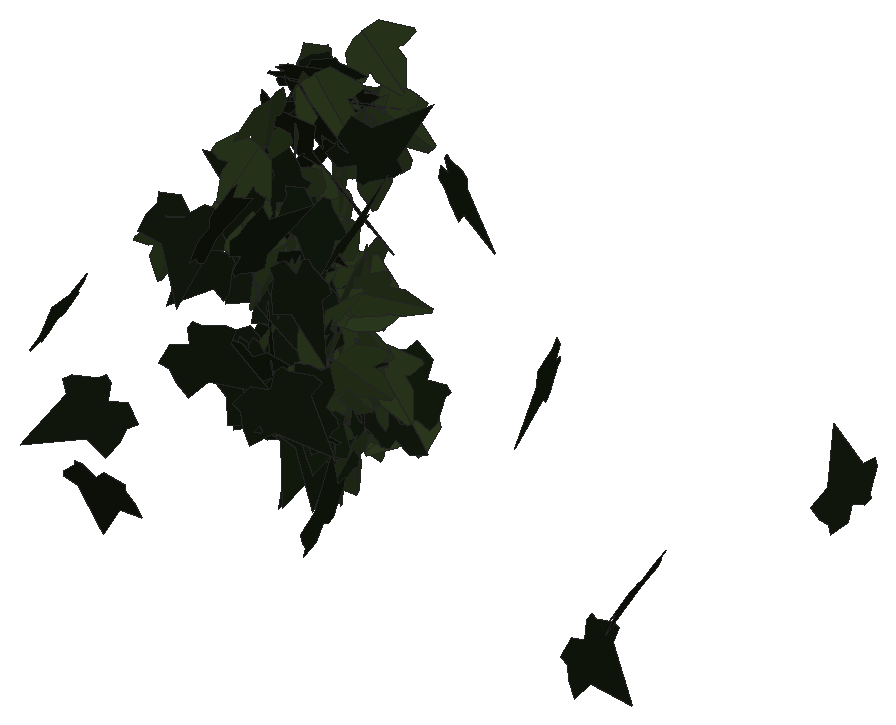
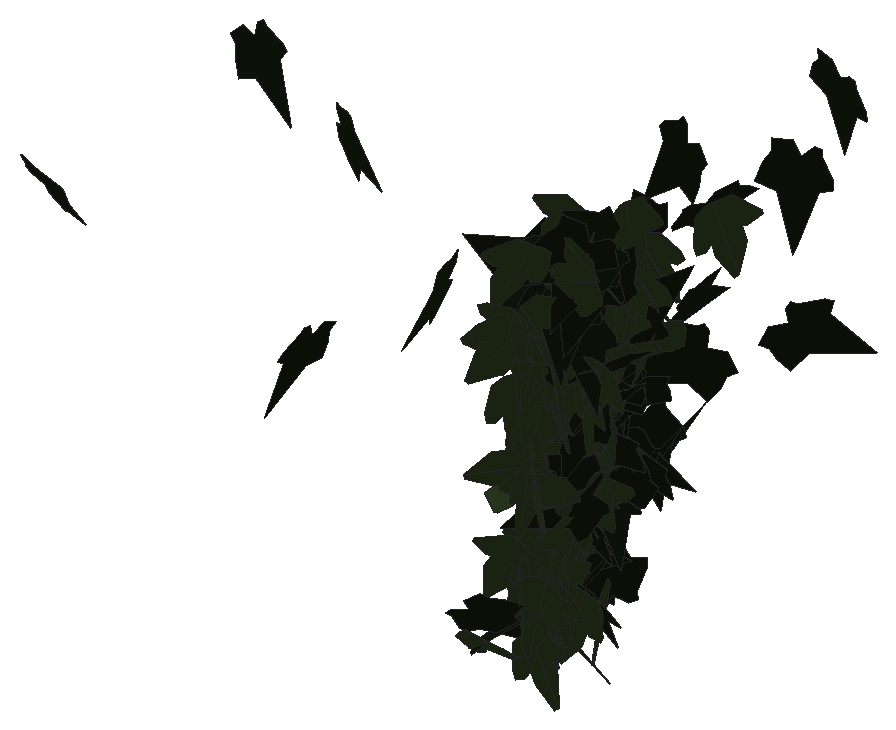
# SketchUp Ruby script. Lengths in inches.
U = 1.inch
M = Sketchup.active_model
def pt(a) = Geom::Point3d.new(a.map { |v| v * U })
def face(e, loops, mat)
  f = e.add_face(loops[0].map { |a| pt(a) })
  loops[1..].each { |l| e.add_face(l.map { |a| pt(a) }).erase! }
  f.material = f.back_material = mat if mat
  f
end
# faces: each face lists its corners as indices into pts; further lists are holes
def faces(e, pts, list, mat = nil) = list.each { |f| face(e, (f[0].is_a?(Array) ? f : [f]).map { |l| l.map { |i| pts[i] } }, mat) }
# xy, xz, yz: faces in a plane at the given z, y or x. An outline is a flat list of corners, or four numbers for a rectangle; further outlines are holes
def ring(l) = l.size == 4 ? [[l[0], l[1]], [l[2], l[1]], [l[2], l[3]], [l[0], l[3]]] : l.each_slice(2).to_a
def flat(e, list, mat, &to3) = list.each { |f| face(e, (f[0].is_a?(Array) ? f : [f]).map { |l| ring(l).map { |u, v| to3.(u, v) } }, mat) }
def xy(e, z, list, mat = nil) = flat(e, list, mat) { |x, y| [x, y, z] }
def xz(e, y, list, mat = nil) = flat(e, list, mat) { |x, z| [x, y, z] }
def yz(e, x, list, mat = nil) = flat(e, list, mat) { |y, z| [x, y, z] }
def lines(e, pts, list) = list.each { |a, b| e.add_line(pt(pts[a]), pt(pts[b])) }
# prism: a flat outline (further loops are holes) pulled along v
def prism(e, loops, v, mat = nil)
  f = face(e, loops, mat); d = Geom::Vector3d.new(v.map { |x| x * U })
  f.pushpull(f.normal.samedirection?(d) ? d.length : -d.length)
end
def box(e, o, s, mat = nil) = prism(e, [[o, [o[0] + s[0], o[1], o[2]], [o[0] + s[0], o[1] + s[1], o[2]], [o[0], o[1] + s[1], o[2]]]], [0, 0, s[2]], mat)
def at(x, y, z, deg = 0) = Geom::Transformation.translation(pt([x, y, z])) * Geom::Transformation.rotation(ORIGIN, Z_AXIS, deg.degrees)
def axes(o, x, y, z) = Geom::Transformation.new([*x, 0, *y, 0, *z, 0, *pt(o).to_a, 1])
def part(name) = M.definitions.add(name)
# library, detail: a bought-in or finely detailed component or shape, given as its bounding box
def library(name, o, s) = part(name).tap { |d| box(d.entities, o, s) }
def detail(e, o, s) = box(e.add_group.entities, o, s)
def put(e, d, t, mat = nil) = e.add_instance(d, t).tap { |i| i.material = mat if mat }
def group(e, t, mat = nil) = e.add_group.tap { |g| g.transformation = t; g.material = mat if mat }.entities
root = M.entities
M.materials.add("efeu1").color = [18, 25, 13]
M.materials.add("efeu2").color = [43, 57, 29]
c1 = part("ivyleaf_10")
p = [[0,0.5,-0.03],[-0.0625,2.02,-0.43],[-0.19,2.01,-0.46],[-0.54,1.05,-0.29],[-0.52,0.625,-0.18],[-0.83,0.76,-0.28],
  [-1.16,0.64,-0.33],[-1.15,0.33,-0.24],[-0.77,-0.39,0.02],[-0.3,-0.51,0.16],[0.04,-0.48,0.23],[-0.02,2.01,-0.4375],
  [-0.06,2.01,-0.43],[0.04,-0.49,0.23],[0.67,-0.49,0.14],[1.38,0.36,-0.2],[1.375,0.51,-0.24],[0.81,0.65,-0.19],
  [0.62,0.59,-0.15],[0.6,1.09,-0.28],[0.5,1.23,-0.31]]
faces(c1.entities,p,[[0,1,2,3,4,5,6,7,8,9,10],[11,12,0,13,14,15,16,17,18,19,20]],"efeu2")
c2 = part("ivyleaf_9")
p = [[1.54,2.16,1.25],[1.36,2.04,1.19],[-0.21,0.99,0.68],[-0.71,1.11,0.82],[-0.85,0.86,0.67],[-0.8,0.17,0.21],
  [-0.9,-0.01,0.1],[-0.67,-0.16,-0.02],[-0.08,-0.08,-0.05],[-0.03,-0.6,-0.4],[0.65,-0.88,-0.66],[0.83,-0.6,-0.49],
  [1.29,-0.42,-0.43],[1.8125,-0.07,-0.26],[1.21,0.44,0.15]]
faces(c2.entities,p,[[0,1,2,3,4,5,6,7,8,9,10,11,12,13,14]],"efeu1")
put(root,c1,axes([54.52,225.38,209.37],[0.06794,0.47554,0.13874],[-0.053,0.14622,-0.4752],[-0.49252,0.04986,0.07027]))
put(root,c2,axes([54.43,224.8,212.04],[-0.17029,-0.46723,0.05192],[0.09679,-0.08888,-0.48242],[0.46004,-0.15425,0.12071]))
put(root,c1,axes([54.47,224.94,211.95],[-0.46815,-0.03134,-0.17279],[0.17195,-0.18173,-0.43291],[-0.03567,-0.46475,0.18093]))
put(root,c1,axes([54.58,224.75,211.125],[0.07251,-0.48194,0.11169],[0.03199,-0.10808,-0.48713],[0.49368,0.07778,0.01516]))
put(root,c1,axes([54.57,224.875,209.74],[0.11655,0.09989,-0.47586],[0.0633,0.48205,0.1167],[0.48209,-0.08745,0.09972]))
put(root,c2,axes([54.8,219.61,210.4],[-0.01506,-0.06036,-0.49611],[-0.11412,-0.48281,0.06221],[-0.48657,0.11511,0.00076]))
put(root,c1,axes([54.61,223.75,213.02],[-0.18239,-0.43215,-0.17316],[0.0597,0.16273,-0.46899],[0.4617,-0.19175,-0.00776]))
put(root,c1,axes([54.76,224.34,207.58],[-0.23006,0.25819,0.36112],[-0.24578,0.26463,-0.34578],[-0.36969,-0.33661,0.00515]))
put(root,c2,axes([54.84,223.76,212.22],[0.08417,0.02553,0.4922],[-0.48104,-0.10448,0.08767],[0.10733,-0.48829,0.00697]))
put(root,c1,axes([54.66,224.65,209.55],[-0.47194,0.16379,0.02103],[-0.0203,0.00564,-0.49956],[-0.16388,-0.47238,0.00132]))
put(root,c2,axes([54.83,224.15,209.55],[-0.10043,0.48531,0.06627],[-0.03715,0.05991,-0.49501],[-0.4884,-0.10435,0.02402]))
put(root,c1,axes([54.67,226.05,208.43],[-0.49533,0.06801,0.00507],[-0.00501,0.00076,-0.49997],[-0.06801,-0.49535,-0.00007]))
put(root,c1,axes([54.95,225.86,207.34],[-0.39652,0.03395,0.30269],[-0.30458,-0.04808,-0.3936],[0.00238,-0.49652,0.05881]))
put(root,c2,axes([54.87,224.76,212.64],[-0.07203,0.48635,-0.09095],[0.01821,-0.08924,-0.49163],[-0.49445,-0.07413,-0.00485]))
put(root,c2,axes([54.4,225.17,209.96],[0.44623,0.05922,0.21766],[0.20549,0.09228,-0.44638],[-0.09304,0.48783,0.05802]))
put(root,c1,axes([54.73,225.03,207.79],[-0.49219,0.06307,-0.06142],[0.06021,-0.01334,-0.49618],[-0.06423,-0.49583,0.00554]))
put(root,c1,axes([54.85,225.43,212.1],[0.29412,-0.27482,-0.29659],[-0.15217,0.26457,-0.39604],[0.37462,0.32323,0.07199]))
put(root,c2,axes([54.62,224.63,211.08],[-0.07419,-0.47381,0.14143],[0.00295,-0.14344,-0.47897],[0.49446,-0.07024,0.02407]))
put(root,c2,axes([54.97,224.75,213.92],[-0.45932,0.18416,-0.07144],[0.05499,-0.05447,-0.49397],[-0.18973,-0.46165,0.02979]))
put(root,c1,axes([54.89,224.2,212.43],[-0.32114,-0.36465,0.11788],[-0.08489,-0.08229,-0.48582],[0.37371,-0.33205,-0.00906]))
put(root,c2,axes([54.82,224.61,213.58],[0.20655,0.45525,0.00906],[-0.01589,0.01715,-0.49945],[-0.45507,0.20603,0.02155]))
put(root,c1,axes([54.4,225.23,213.76],[0.1666,-0.04389,0.46938],[0.46109,0.11885,-0.15255],[-0.09818,0.48368,0.08008]))
put(root,c1,axes([54.8125,224.56,209.5],[0.35481,0.28865,-0.20197],[-0.15364,-0.13117,-0.45737],[-0.31703,0.38662,-0.00438]))
put(root,c1,axes([54.64,223.17,211.71],[0.40941,0.21968,-0.18472],[0.15871,0.09485,0.46456],[0.23915,-0.43902,0.00794]))
put(root,c2,axes([54.75,224.75,214.06],[0.36592,0.33395,-0.06766],[-0.05816,-0.03662,-0.49525],[-0.33574,0.37032,0.01204]))
put(root,c2,axes([54.78,222.39,211.87],[-0.11686,-0.34989,0.33753],[-0.10499,-0.32079,-0.36888],[0.47468,-0.15709,0.0015]))
put(root,c1,axes([54.9,225.94,212.71],[0.32854,-0.32036,-0.19857],[-0.13105,0.14989,-0.45865],[0.35339,0.35341,0.01452]))
put(root,c2,axes([54.75,224.6875,211.21],[0.44782,0.06128,-0.21378],[-0.21253,-0.02358,-0.45197],[-0.06548,0.49567,0.00493]))
put(root,c1,axes([54.8,225.26,208.74],[-0.26541,0.42194,0.03898],[-0.02423,0.03081,-0.49846],[-0.42305,-0.26649,0.00409]))
put(root,c1,axes([54.91,223.07,213.28],[0.45298,-0.04054,-0.20775],[-0.20571,0.03131,-0.45464],[0.04987,0.49737,0.01168]))
put(root,c1,axes([54.71,223.3,211.71],[-0.20308,0.42828,-0.15918],[0.08342,-0.13651,-0.47372],[-0.44922,-0.21896,-0.01601]))
put(root,c1,axes([54.83,225.09,209.67],[0.12058,-0.47755,0.08608],[0.02491,-0.08248,-0.49252],[0.4846,0.12306,0.0039]))
put(root,c1,axes([54.8,225.63,208.28],[0.4889,-0.0992,-0.03368],[-0.03257,0.00885,-0.49886],[0.09957,0.48998,0.0022]))
put(root,c1,axes([54.81,225.22,209],[-0.21038,0.4491,0.06363],[-0.01758,0.06201,-0.49583],[-0.45324,-0.21086,-0.0103]))
put(root,c2,axes([54.5625,224.52,214.04],[0.45978,0.08416,0.17754],[0.14322,0.16576,-0.44946],[-0.13451,0.46416,0.12831]))
put(root,c2,axes([54.97,223.29,212.92],[-0.44086,0.13777,-0.19148],[0.18089,-0.06304,-0.46185],[-0.1514,-0.47649,0.00574]))
put(root,c2,axes([54.64,223.98,209.12],[-0.02962,-0.10352,0.48827],[0.4406,0.2244,0.0743],[-0.23452,0.43466,0.07792]))
put(root,c1,axes([55.03,224.05,210.9375],[0.12643,-0.15608,-0.45788],[-0.21162,0.40773,-0.19741],[0.43501,0.24371,0.03704]))
put(root,c2,axes([54.91,223.11,209.21],[0.05359,-0.48467,-0.11057],[0.07854,-0.10156,0.48324],[-0.49088,-0.06916,0.06525]))
put(root,c2,axes([54.6875,225,209.39],[-0.27496,-0.10844,-0.40329],[0.39859,0.07591,-0.29217],[0.1246,-0.48216,0.0447]))
put(root,c2,axes([54.99,225.04,213.26],[0.06704,0.49444,-0.03222],[-0.02102,-0.02965,-0.49868],[-0.49504,0.06822,0.01681]))
put(root,c1,axes([54.92,223.5,213.95],[-0.01631,-0.49588,-0.06193],[0.00752,0.06171,-0.49612],[0.49968,-0.01711,0.00544]))
put(root,c1,axes([54.9375,225.97,212.65],[-0.44945,0.21598,0.03667],[-0.04834,-0.01613,-0.4974],[-0.21368,-0.45066,0.03538]))
put(root,c2,axes([55.3,222.86,209.4375],[-0.23722,-0.04206,-0.43813],[-0.4248,-0.1084,0.24041],[-0.11521,0.48629,0.01569]))
put(root,c1,axes([54.65,224.89,211.53],[0.37298,-0.1544,0.29503],[0.28534,-0.08017,-0.40268],[0.17165,0.46876,0.0283]))
put(root,c2,axes([54.95,224.7,207.85],[-0.45157,-0.05151,-0.2084],[0.21004,-0.00579,-0.45371],[0.04433,-0.49731,0.02686]))
put(root,c2,axes([54.71,224.23,207.72],[0.48596,0.09163,0.07379],[-0.08141,0.03547,0.49205],[0.08493,-0.49025,0.0494]))
put(root,c1,axes([54.85,225.49,208.82],[-0.41659,0.18823,-0.20254],[0.0998,-0.23919,-0.42758],[-0.25786,-0.39668,0.16172]))
put(root,c2,axes([54.93,224.51,209.19],[-0.31646,0.38592,0.03026],[0.01328,-0.02824,0.49903],[0.38688,0.31665,0.00762]))
put(root,c2,axes([54.73,223.71,211.08],[-0.03486,-0.41639,-0.27459],[0.07825,0.26729,-0.41525],[0.49261,-0.07192,0.04653]))
put(root,c1,axes([55.02,221.17,212.9],[-0.17869,-0.44916,0.12778],[-0.04968,-0.11776,-0.48339],[0.46433,-0.18545,-0.00255]))
put(root,c1,axes([55.01,225.85,213.13],[-0.07137,-0.44036,0.2258],[-0.03247,-0.22348,-0.4461],[0.49381,-0.07834,0.00331]))
put(root,c1,axes([54.76,224.58,213.74],[0.1898,-0.29467,0.35657],[0.26038,-0.25051,-0.34561],[0.38233,0.31688,0.05836]))
put(root,c2,axes([54.65,224.34,213.06],[-0.07762,-0.14291,0.47281],[0.33212,-0.36937,-0.05712],[0.36561,0.30519,0.15227]))
put(root,c1,axes([55.08,225.0625,207],[0.13516,-0.09294,-0.47233],[-0.12053,0.46843,-0.12667],[0.46605,0.1481,0.10422]))
put(root,c1,axes([54.96,225.68,210.04],[0.2168,-0.44611,0.06309],[0.0493,-0.04611,-0.49542],[0.44785,0.22103,0.02399]))
put(root,c2,axes([54.81,223.5,209.75],[-0.2502,-0.20157,-0.38311],[0.35177,0.16323,-0.31561],[0.25231,-0.42746,0.06013]))
put(root,c2,axes([54.86,224.04,211.38],[0.14289,-0.271,-0.39515],[-0.1064,0.3841,-0.3019],[0.46718,0.17036,0.05211]))
put(root,c1,axes([54.92,225.7,210.17],[0.45355,0.21046,0.00141],[0.00504,-0.00751,-0.49992],[-0.2104,0.45349,-0.00893]))
put(root,c1,axes([55.08,226.12,211.97],[-0.24425,-0.43505,0.03271],[-0.00999,-0.03191,-0.49888],[0.43617,-0.24436,0.0069]))
put(root,c1,axes([55.03,223.7,211.39],[0.02571,-0.40259,0.2954],[0.04101,-0.29309,-0.40301],[0.49765,0.04495,0.01795]))
put(root,c2,axes([55.34,225.02,207.43],[-0.42675,0.22585,0.12993],[-0.1125,0.06518,-0.4828],[-0.23502,-0.4413,-0.00482]))
put(root,c1,axes([55.03,223.9,209.83],[-0.13233,-0.48136,0.02803],[0.07303,-0.04874,-0.49223],[0.47661,-0.12618,0.08321]))
put(root,c2,axes([55.01,223.73,211.44],[0.23516,0.43357,0.08198],[0.0385,0.07237,-0.49323],[-0.43957,0.23829,0.00065]))
put(root,c2,axes([55.2,223.22,210.1875],[0.14373,-0.01598,-0.47863],[-0.45434,0.15343,-0.14156],[0.15139,0.47561,0.02958]))
put(root,c2,axes([54.85,224.28,210.42],[-0.22745,-0.26818,-0.35545],[0.27799,0.22628,-0.3486],[0.34784,-0.3562,0.04617]))
put(root,c1,axes([54.9,223.92,211.6],[-0.26686,0.27959,-0.3172],[0.1861,-0.25915,-0.38498],[-0.37968,-0.32353,0.03425]))
put(root,c1,axes([55.11,224.98,211.2],[-0.19924,-0.38088,0.25541],[0.02548,-0.28724,-0.40847],[0.45788,-0.14975,0.13387]))
put(root,c1,axes([55.02,225.72,208.51],[-0.41909,0.25832,-0.08738],[0.07069,-0.05181,-0.49226],[-0.26337,-0.42496,0.0069]))
put(root,c1,axes([55.04,225.25,211.46],[0.39202,-0.30818,0.03669],[0.02039,-0.03341,-0.49847],[0.30968,0.39231,-0.01362]))
put(root,c1,axes([55.08,225.77,210.28],[0.01169,-0.46826,-0.17491],[0.0782,0.17451,-0.46198],[0.49371,-0.01655,0.07732]))
put(root,c1,axes([55.18,224.46,209.38],[-0.12763,-0.48025,0.05542],[-0.01449,-0.05349,-0.49692],[0.48322,-0.12845,-0.00026]))
put(root,c2,axes([55.25,222.74,209.95],[0.2641,0.22552,-0.35971],[-0.26863,-0.23928,-0.34725],[-0.32877,0.37668,-0.00522]))
put(root,c1,axes([54.95,224.67,210.13],[0.1162,0.28865,0.39138],[0.13333,0.36807,-0.31104],[-0.46767,0.17665,0.00857]))
put(root,c1,axes([55.16,225.8,208.51],[0.16281,-0.44362,-0.16338],[-0.00709,0.17048,-0.46998],[0.4727,0.15536,0.04922]))
put(root,c1,axes([54.94,225.42,207.52],[0.23982,-0.28653,0.33225],[0.26323,-0.20896,-0.3702],[0.351,0.35248,0.05062]))
put(root,c2,axes([55.13,224.45,208.09],[-0.2872,-0.40858,-0.02409],[0.01363,0.01987,-0.49942],[0.40906,-0.28753,-0.00028]))
put(root,c1,axes([55.08,224.59,208.28],[0.049,-0.25315,0.42839],[-0.0197,0.42914,0.25584],[-0.4972,-0.04195,0.03208]))
put(root,c2,axes([55.0625,223.62,211.22],[0.40004,0.29736,-0.03932],[-0.02721,-0.02929,-0.4984],[-0.29871,0.4009,-0.00725]))
put(root,c2,axes([54.97,224.59,207.89],[0.05334,-0.48593,0.10501],[0.00301,-0.1053,-0.48878],[0.49714,0.05278,-0.00831]))
put(root,c1,axes([54.89,224.4,209.87],[0.10362,0.08147,-0.48231],[0.368,0.3118,0.13173],[0.32224,-0.38228,0.00465]))
put(root,c1,axes([55.08,223.94,211.45],[0.39691,-0.2956,0.07128],[0.06189,-0.03621,-0.49483],[0.29771,0.40163,0.00785]))
put(root,c1,axes([55.21,225.78,208.09],[0.4483,-0.18136,-0.12702],[-0.11002,0.06646,-0.4832],[0.19215,0.46119,0.01969]))
put(root,c1,axes([55.17,224.02,210.58],[0.1478,0.46048,-0.12692],[0.0335,0.12254,0.48359],[0.47648,-0.15146,0.00537]))
put(root,c1,axes([55.0625,223.91,209.64],[0.48596,0.105,0.05307],[0.04223,0.05483,-0.49519],[-0.10981,0.48577,0.04442]))
put(root,c1,axes([55.11,225.03,209.5],[0.00507,0.49819,-0.04218],[-0.00417,-0.04214,-0.4982],[-0.49996,0.00541,0.00373]))
put(root,c1,axes([55.16,225.5,209.08],[-0.45391,0.19524,-0.07647],[0.07089,-0.02872,-0.49412],[-0.19734,-0.45941,-0.00161]))
put(root,c2,axes([54.79,224.42,213.67],[0.20905,0.04045,-0.4524],[0.45064,0.04378,0.21215],[0.05677,-0.49643,-0.01816]))
put(root,c1,axes([55.27,225.36,210.44],[0.19003,-0.46226,-0.01446],[-0.00449,0.01378,-0.49979],[0.46246,0.19008,0.00109]))
put(root,c1,axes([55.16,225.5,209.06],[-0.46168,0.08891,-0.17014],[0.16075,-0.06318,-0.46922],[-0.10494,-0.48796,0.02975]))
put(root,c1,axes([55.33,224.53,209.48],[0.22313,-0.44169,-0.07156],[-0.04038,0.05977,-0.49477],[0.44562,0.22658,-0.009]))
put(root,c2,axes([55.18,221.23,213.13],[-0.11717,-0.48569,-0.01948],[0.00514,0.0188,-0.49962],[0.48605,-0.11728,0.00059]))
put(root,c1,axes([55.03,223.76,211.78],[0.39939,0.14523,0.26343],[0.25068,0.08135,-0.4249],[-0.16628,0.47148,-0.00783]))
put(root,c1,axes([55.67,225.5,209.71],[-0.0065,0.49807,0.04345],[-0.48086,-0.01812,0.13581],[0.13686,-0.04002,0.47924]))
put(root,c2,axes([55.18,224.74,213.69],[0.46307,0.18385,0.04199],[-0.05013,0.22734,-0.4425],[-0.1818,0.40561,0.22898]))
put(root,c1,axes([55.16,225.78,214.18],[0.19522,0.38073,0.25871],[0.0916,0.24326,-0.42712],[-0.45111,0.21416,0.02523]))
put(root,c1,axes([55.35,225.04,207.3],[0.02911,-0.46784,-0.174],[0.02144,0.17531,-0.46777],[0.49869,0.01978,0.03026]))
put(root,c1,axes([54.98,225.23,208.4],[-0.03844,0.01087,-0.4984],[0.41562,-0.27534,-0.03806],[-0.27529,-0.41722,0.01213]))
put(root,c1,axes([55.2,226.07,212.87],[-0.32965,-0.20223,-0.31691],[0.28113,0.14722,-0.38638],[0.24959,-0.43293,0.01664]))
put(root,c2,axes([55.69,225.71,207.43],[-0.07569,0.49414,0.00976],[-0.4902,-0.07631,0.06231],[0.06307,-0.00014,0.49601]))
put(root,c1,axes([55.62,226.41,207.48],[-0.41734,0.18698,0.20214],[-0.25996,-0.38858,-0.17727],[0.09081,-0.25306,0.42156]))
put(root,c2,axes([55.07,221.47,210.67],[0.03376,-0.02488,-0.49824],[0.24286,0.43702,-0.00537],[0.43575,-0.24164,0.0416]))
put(root,c2,axes([55.625,226.51,208.04],[-0.43262,-0.20909,0.13827],[-0.1229,-0.06346,-0.48049],[0.21848,-0.44973,0.00351]))
put(root,c1,axes([55.1875,226.0625,212.97],[-0.24297,-0.01467,-0.43675],[0.43467,-0.05957,-0.23982],[-0.045,-0.49622,0.0417]))
put(root,c2,axes([55.17,225.05,211.9],[0.30522,-0.29297,0.26647],[0.19795,-0.17853,-0.42302],[0.34301,0.36372,0.007]))
put(root,c2,axes([55.8,217.17,213.31],[-0.08709,0.43116,0.23774],[-0.07305,0.22744,-0.43924],[-0.48691,-0.11124,0.02337]))
put(root,c1,axes([55.4,224.24,214.14],[0.36484,0.17689,0.29258],[0.24885,0.15601,-0.40464],[-0.23445,0.44087,0.0258]))
put(root,c1,axes([55.5,225.53,208.66],[0.33431,0.25278,0.27266],[0.21656,0.16567,-0.41911],[-0.30222,0.39832,0.00129]))
put(root,c2,axes([55.58,223.83,212.27],[0.06894,-0.49366,0.03929],[0.00229,-0.03935,-0.49844],[0.49522,0.06891,-0.00317]))
put(root,c1,axes([55.52,225.23,210.07],[0.12779,-0.06778,0.47862],[0.34878,0.3557,-0.04276],[-0.33469,0.34479,0.13819]))
put(root,c2,axes([55.62,224.65,209.05],[-0.20148,-0.45754,0.00786],[0.45196,-0.2003,-0.07489],[0.07167,-0.02307,0.4943]))
put(root,c2,axes([55.85,221.78,212.47],[0.0966,0.13203,0.47248],[0.2931,0.37063,-0.16349],[-0.3934,0.30855,-0.00579]))
put(root,c2,axes([56.12,220.61,213.55],[-0.12329,0.17216,-0.45294],[-0.28183,0.35471,0.21154],[0.39417,0.30747,0.00958]))
put(root,c2,axes([56.35,223.1,207.3],[-0.33221,0.21421,-0.30619],[-0.26759,0.1496,0.39499],[0.26083,0.4263,0.01525]))
put(root,c2,axes([56.03,224.42,213],[-0.02225,-0.03046,0.49857],[0.45876,0.19617,0.03246],[-0.19759,0.4589,0.01922]))
put(root,c2,axes([56.13,222.74,211.71],[0.18242,-0.45217,-0.11075],[-0.04438,0.10152,-0.48757],[0.46342,0.18771,-0.00309]))
put(root,c2,axes([56.6,223.28,212.18],[-0.26091,0.37196,-0.20874],[-0.12017,0.17068,0.45434],[0.40925,0.28726,0.00033]))
put(root,c1,axes([56.5,223.51,209.93],[-0.28439,-0.23715,-0.33598],[0.2587,0.21438,-0.37029],[0.31968,-0.38445,0.00077]))
put(root,c2,axes([56.82,222.51,209.76],[-0.12955,-0.21216,0.43382],[-0.23972,-0.36166,-0.24846],[0.41923,-0.27237,-0.00801]))
put(root,c2,axes([56.7,221.41,210.45],[-0.0122,-0.20562,-0.4556],[0.09797,0.44592,-0.20387],[0.49016,-0.09424,0.02941]))
put(root,c2,axes([57.08,216.56,211.17],[0.35945,0.18093,-0.29675],[-0.26851,-0.1265,-0.40237],[-0.22068,0.44862,0.00622]))
put(root,c2,axes([57.18,225.24,212.78],[0.38019,-0.26514,-0.1875],[-0.15364,0.10747,-0.46351],[0.2861,0.41006,0.00024]))
put(root,c2,axes([61.8,221.99,212.47],[-0.36687,0.16296,-0.29808],[0.26333,-0.14076,-0.40105],[-0.21462,-0.45126,0.01745]))
put(root,c2,axes([62.875,221.5,208.14],[0.17361,-0.26799,-0.38476],[-0.19317,0.33297,-0.31908],[0.42725,0.25944,0.01208]))
put(root,c2,axes([65.88,219.08,211.33],[-0.24278,0.41665,-0.13214],[0.06801,-0.11331,-0.48222],[-0.43178,-0.25212,-0.00166]))
put(root,c2,axes([66.2,223.91,210.77],[-0.44388,0.08403,-0.21428],[-0.20976,0.04392,0.45174],[0.09474,0.49093,-0.00374]))
